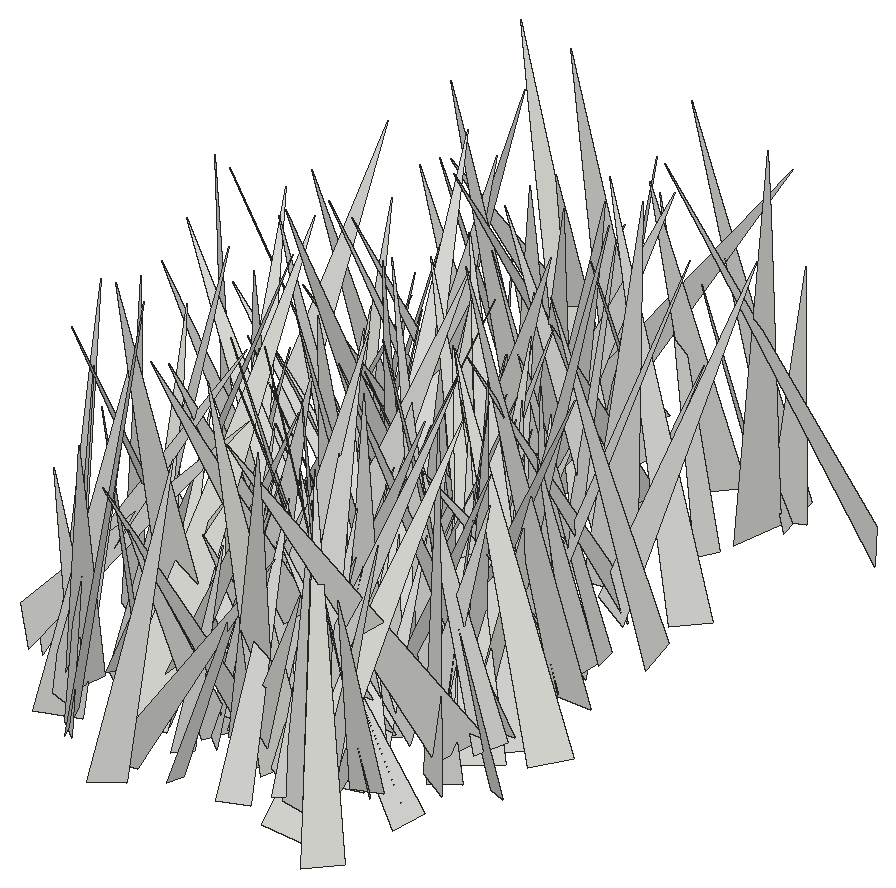
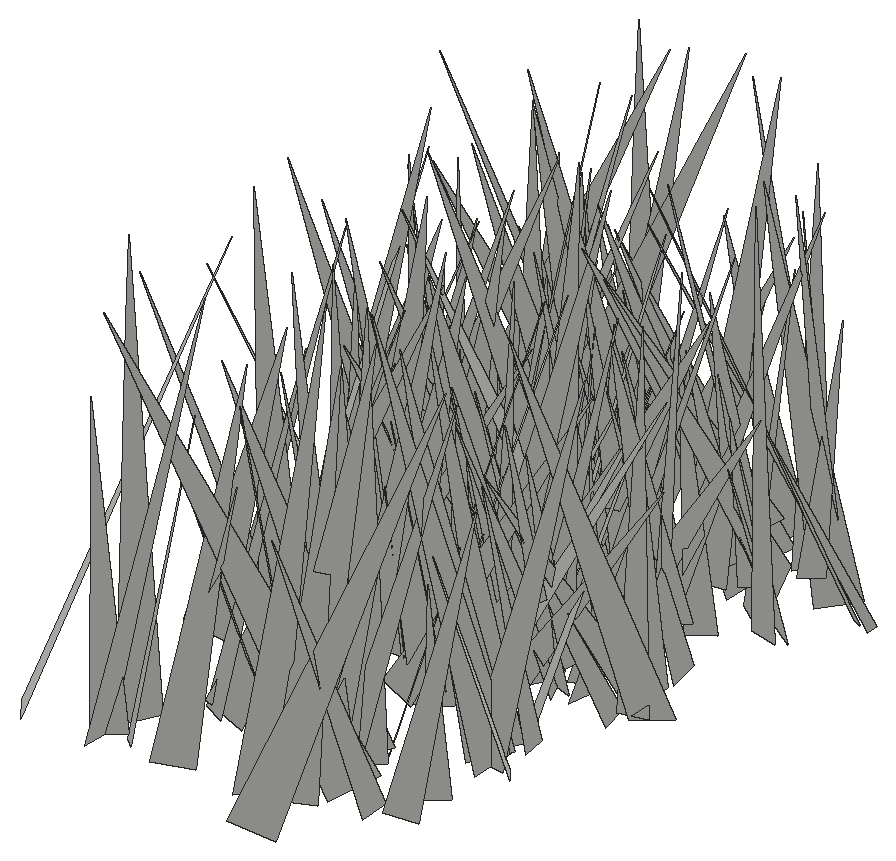
# SketchUp Ruby script. Lengths in inches.
U = 1.inch
M = Sketchup.active_model
def pt(a) = Geom::Point3d.new(a.map { |v| v * U })
def face(e, loops, mat)
  f = e.add_face(loops[0].map { |a| pt(a) })
  loops[1..].each { |l| e.add_face(l.map { |a| pt(a) }).erase! }
  f.material = f.back_material = mat if mat
  f
end
# faces: each face lists its corners as indices into pts; further lists are holes
def faces(e, pts, list, mat = nil) = list.each { |f| face(e, (f[0].is_a?(Array) ? f : [f]).map { |l| l.map { |i| pts[i] } }, mat) }
# xy, xz, yz: faces in a plane at the given z, y or x. An outline is a flat list of corners, or four numbers for a rectangle; further outlines are holes
def ring(l) = l.size == 4 ? [[l[0], l[1]], [l[2], l[1]], [l[2], l[3]], [l[0], l[3]]] : l.each_slice(2).to_a
def flat(e, list, mat, &to3) = list.each { |f| face(e, (f[0].is_a?(Array) ? f : [f]).map { |l| ring(l).map { |u, v| to3.(u, v) } }, mat) }
def xy(e, z, list, mat = nil) = flat(e, list, mat) { |x, y| [x, y, z] }
def xz(e, y, list, mat = nil) = flat(e, list, mat) { |x, z| [x, y, z] }
def yz(e, x, list, mat = nil) = flat(e, list, mat) { |y, z| [x, y, z] }
def lines(e, pts, list) = list.each { |a, b| e.add_line(pt(pts[a]), pt(pts[b])) }
# prism: a flat outline (further loops are holes) pulled along v
def prism(e, loops, v, mat = nil)
  f = face(e, loops, mat); d = Geom::Vector3d.new(v.map { |x| x * U })
  f.pushpull(f.normal.samedirection?(d) ? d.length : -d.length)
end
def box(e, o, s, mat = nil) = prism(e, [[o, [o[0] + s[0], o[1], o[2]], [o[0] + s[0], o[1] + s[1], o[2]], [o[0], o[1] + s[1], o[2]]]], [0, 0, s[2]], mat)
def at(x, y, z, deg = 0) = Geom::Transformation.translation(pt([x, y, z])) * Geom::Transformation.rotation(ORIGIN, Z_AXIS, deg.degrees)
def axes(o, x, y, z) = Geom::Transformation.new([*x, 0, *y, 0, *z, 0, *pt(o).to_a, 1])
def part(name) = M.definitions.add(name)
# library, detail: a bought-in or finely detailed component or shape, given as its bounding box
def library(name, o, s) = part(name).tap { |d| box(d.entities, o, s) }
def detail(e, o, s) = box(e.add_group.entities, o, s)
def put(e, d, t, mat = nil) = e.add_instance(d, t).tap { |i| i.material = mat if mat }
def group(e, t, mat = nil) = e.add_group.tap { |g| g.transformation = t; g.material = mat if mat }.entities
root = M.entities
c1 = part("fur_instance\#9")
p = [[0.8125,0,1.79],[0.67,-0.02,1.48],[0,-0.11,0],[0,0.11,0]]
faces(c1.entities,p,[[0,1,2,3]])
put(root,c1,axes([134.02,205.54,-27.1],[-1.22058,7.14872,1.6543],[7.02907,1.62036,-1.81584],[2.10547,-1.26529,7.02116]))
put(root,c1,axes([134.57,199.46,-27.1],[-2.31612,-6.1908,2.36322],[-6.27799,2.85121,1.3163],[2.12077,1.67923,6.47748]))
put(root,c1,axes([136.18,215.1,-27.1],[1.56838,-4.91392,1.31708],[-4.91027,-1.82266,-0.95305],[-1.33063,0.93404,5.06933]))
put(root,c1,axes([134.63,205.76,-27.1],[-0.27546,-6.0552,1.07535],[-6.00995,0.49341,1.23885],[1.30474,0.99438,5.93351]))
put(root,c1,axes([136.3125,210.85,-27.1],[-0.27695,-6.43694,1.01641],[-6.49492,0.18954,-0.56932],[-0.53231,1.03627,6.4177]))
put(root,c1,axes([135.78,195.63,-27.1],[3.23004,-2.47849,1.2151],[-2.38486,-3.44753,-0.69249],[-1.3899,0.15559,4.01205]))
put(root,c1,axes([138.625,206.86,-27.1],[-4.24155,2.82864,0.08548],[2.61337,3.85608,2.07369],[-1.08573,-1.76881,4.65744]))
put(root,c1,axes([139.25,207.15,-27.1],[-5.24888,-4.54366,0.15791],[-4.36596,4.97023,-2.11085],[-1.26815,1.69482,6.61361]))
put(root,c1,axes([136.17,194.08,-27.1],[2.58836,6.22661,1.98748],[6.38761,-2.86286,0.6503],[-1.38536,-1.56644,6.71174]))
put(root,c1,axes([136.29,196.8,-28.22],[1.50713,3.43781,0.3216],[3.3001,-1.53741,0.96906],[-1.01552,0.10596,3.62641]))
put(root,c1,axes([136.01,213.55,-27.1],[-2.23187,2.81976,1.51549],[3.01775,2.4697,-0.15093],[1.06816,-1.08561,3.59298]))
put(root,c1,axes([136.5,208.49,-27.1],[-3.05725,-3.63504,0.09512],[-3.51202,2.98398,1.15363],[0.94245,-0.67208,4.60753]))
put(root,c1,axes([137.71,200.69,-28.22],[-7.59721,-1.99805,2.32928],[-2.54922,7.5713,-1.81993],[1.70857,2.41215,7.64184]))
put(root,c1,axes([136.1,202.68,-28.22],[4.53301,0.32886,1.81446],[0.26511,-4.88148,0.22244],[-1.82486,0.10775,4.53948]))
put(root,c1,axes([135.27,210.93,-27.1],[2.99336,2.37967,0.42143],[2.41657,-2.95437,-0.48225],[-0.02533,-0.63994,3.79348]))
put(root,c1,axes([137.33,200.68,-27.1],[-3.85678,5.81728,0.33644],[5.7739,3.8696,-0.71896],[0.78484,0.11882,6.94252]))
put(root,c1,axes([136.83,197.25,-27.1],[-1.83169,3.1238,0.57494],[3.14275,1.87858,-0.19441],[0.4602,-0.39568,3.61599]))
put(root,c1,axes([135.76,209.14,-27.1],[4.33952,0.70183,1.00017],[0.70812,-4.45199,0.05164],[-0.99573,-0.10739,4.3956]))
put(root,c1,axes([137.8,204.35,-28.22],[-7.13222,-2.21187,1.52983],[-1.72076,7.08542,2.22194],[2.06682,-1.73369,7.12909]))
put(root,c1,axes([135.28,194.89,-28.22],[4.4224,-5.22883,1.99199],[-5.58659,-4.26873,1.19762],[-0.31423,2.30295,6.7427]))
put(root,c1,axes([135.56,204.58,-27.1],[4.79921,1.03907,0.41248],[0.79797,-4.45725,1.94381],[-0.78297,1.82633,4.50929]))
put(root,c1,axes([132.9375,196.93,-27.1],[5.32286,5.30667,0.20638],[4.93366,-4.8331,-2.97258],[1.96528,-2.23975,6.90343]))
put(root,c1,axes([132.29,197.01,-27.1],[4.7067,5.43888,0.18038],[4.50837,-3.76361,-4.15655],[3.04771,-2.83211,5.87006]))
put(root,c1,axes([137.07,197.03,-28.22],[-3.25628,-4.53556,1.56998],[-4.60157,3.48952,0.53691],[1.36443,0.94415,5.55755]))
put(root,c1,axes([136.23,201.25,-28.22],[5.06172,0.87175,1.3003],[0.68802,-5.19178,0.80241],[-1.40619,0.59773,5.07318]))
put(root,c1,axes([135.62,197.36,-28.22],[-3.45696,-5.56122,4.74392],[-6.59951,4.63089,0.61955],[3.14299,3.60698,6.51874]))
put(root,c1,axes([139.35,199.17,-27.1],[-2.95637,3.32548,0.26078],[3.10336,2.61427,1.84435],[-1.22309,-1.40488,4.04936]))
put(root,c1,axes([138.59,199.73,-28.22],[-3.06964,-6.81398,0.3454],[-6.81954,3.05272,-0.38339],[-0.20825,0.47214,7.46364]))
put(root,c1,axes([137.68,205.73,-27.1],[0.92539,5.82013,0.73982],[5.78512,-1.02986,0.86568],[-0.97656,-0.58571,5.82931]))
put(root,c1,axes([137.36,192.82,-27.1],[3.68214,4.39884,2.0354],[4.4735,-4.06815,0.69917],[-1.86561,-1.07294,5.69378]))
put(root,c1,axes([136.18,196.54,-27.1],[6.68377,2.4417,1.0502],[1.89436,-6.36953,2.75283],[-1.86446,2.28139,6.56175]))
put(root,c1,axes([138.0625,195.86,-27.1],[-5.38629,2.97439,0.98855],[2.72826,5.41671,-1.43257],[1.54299,0.80541,5.98388]))
put(root,c1,axes([138.54,205.72,-27.1],[-6.31827,-0.38458,1.65434],[-0.20418,6.49842,0.73085],[1.68614,-0.65417,6.28763]))
put(root,c1,axes([136.23,204.65,-28.22],[4.0884,0.15219,0.34801],[0.0557,-3.96154,1.07814],[-0.37573,1.0688,3.94662]))
put(root,c1,axes([136.04,195.26,-27.1],[5.72206,-2.67718,0.30846],[-2.55509,-5.6197,-1.37653],[-0.85672,-1.12072,6.16558]))
put(root,c1,axes([135.36,198.06,-27.1],[3.3764,2.66955,0.1135],[2.47122,-3.05035,-1.76859],[1.01611,-1.452,3.92412]))
put(root,c1,axes([138.07,204.73,-27.1],[3.76541,-0.98312,2.37268],[-1.72485,-4.08783,1.04352],[-1.9029,1.75998,3.74912]))
put(root,c1,axes([137.4,198.97,-28.22],[2.1664,-3.98299,1.68795],[-4.30586,-2.16689,0.41322],[-0.41582,1.68731,4.51516]))
put(root,c1,axes([141.62,200.76,-27.1],[-4.54084,5.90887,0.08971],[5.53212,4.21055,2.68494],[-2.07809,-1.7025,6.95162]))
put(root,c1,axes([136.06,210.7,-27.1],[7.69259,-0.4984,1.40276],[-0.64413,-7.77059,0.77146],[-1.3421,0.87272,7.67002]))
put(root,c1,axes([136.43,210.43,-27.1],[4.89354,-4.52263,1.72188],[-4.82903,-4.72322,1.31813],[-0.31551,2.14541,6.53173]))
put(root,c1,axes([137.6,205.68,-27.1],[5.0446,1.96996,1.21492],[1.59207,-5.06819,1.60732],[-1.6799,1.1124,5.17158]))
put(root,c1,axes([138.51,195.8125,-27.1],[-1.52341,4.48001,0.30788],[4.47725,1.54034,-0.26007],[0.34571,-0.20714,4.72479]))
put(root,c1,axes([137.13,193.25,-27.1],[6.97385,3.06548,2.09729],[3.25235,-7.19468,-0.2986],[-1.79388,-1.12684,7.61201]))
put(root,c1,axes([138.26,197.97,-27.1],[1.76512,-7.95634,1.31885],[-8.03843,-1.84494,-0.37166],[-0.65291,1.20466,8.14131]))
put(root,c1,axes([140.49,203.86,-27.1],[-3.6362,-3.51378,0.23491],[-3.4583,3.49912,-1.19165],[-0.6648,1.01649,4.91412]))
put(root,c1,axes([139.24,210.65,-27.1],[-5.93761,-4.29126,0.84113],[-3.95201,5.87307,2.0655],[1.8719,-1.21235,7.02879]))
put(root,c1,axes([138.58,206.69,-27.1],[-1.9531,-3.93926,0.49775],[-3.87343,2.01224,0.72636],[0.87298,0.11511,4.33645]))
put(root,c1,axes([139.25,218.57,-27.1],[4.10096,-6.21113,0.1393],[-5.64172,-3.79303,-3.03306],[-2.60165,-1.56533,6.79681]))
put(root,c1,axes([138.375,203.6,-28.22],[-6.90134,-2.30385,2.57209],[-0.73953,6.60101,3.92832],[3.37291,-3.26662,6.12409]))
put(root,c1,axes([139.78,213.17,-27.1],[-2.67742,-5.68655,1.10676],[-5.79247,2.6077,-0.61446],[-0.09527,1.2623,6.25523]))
put(root,c1,axes([138.95,212.18,-27.1],[-5.78164,-4.6449,0.78576],[-4.06196,5.54542,2.89287],[2.386,-1.8147,6.82889]))
put(root,c1,axes([138.86,194.42,-27.1],[-6.04626,5.73242,0.3376],[5.11125,5.59588,-3.47751],[2.61721,2.31459,7.57131]))
put(root,c1,axes([137.07,215.3,-27.1],[4.6922,-0.3007,0.23761],[-0.32477,-4.66947,0.50417],[-0.20347,0.51889,4.67471]))
put(root,c1,axes([141.125,209.13,-27.1],[-0.84326,-5.89202,0.02664],[-5.53518,0.78295,-2.04363],[-2.01949,0.3143,5.59022]))
put(root,c1,axes([139.04,207.97,-27.1],[0.62863,-8.27068,0.12443],[-8.26435,-0.63324,-0.33804],[-0.34653,0.09834,8.28764]))
put(root,c1,axes([138.26,202.73,-28.22],[-1.07299,-3.39329,1.1863],[-3.30809,1.41653,1.05972],[1.4065,0.74301,3.39746]))
put(root,c1,axes([138.25,206.04,-27.1],[-2.58112,4.19595,2.18678],[4.13957,3.20902,-1.27135],[2.29171,-1.07069,4.75939]))
put(root,c1,axes([140.04,213.76,-27.1],[0.54062,-3.9189,1.26852],[-4.01221,-0.79056,-0.73238],[-0.93225,1.12979,3.88763]))
put(root,c1,axes([137.96,201.32,-27.1],[3.51302,-4.23345,1.0034],[-4.35037,-3.40123,0.88101],[0.05668,1.33409,5.43021]))
put(root,c1,axes([136.41,209.7,-27.1],[0.97454,-6.53217,0.4424],[-5.83998,-0.6651,3.04417],[2.95966,0.83851,5.86106]))
put(root,c1,axes([138.9,206.95,-27.1],[-1.97091,-5.99186,1.73382],[-5.97714,2.33419,1.27215],[1.7839,1.20092,6.17807]))
put(root,c1,axes([141.62,213.34,-27.1],[-4.16616,6.68617,2.08588],[7.00105,3.90518,1.46546],[-0.20279,-2.54114,7.74043]))
put(root,c1,axes([139.93,196.93,-28.22],[2.83348,-4.00549,0.52306],[-3.76222,-2.8494,-1.43972],[-1.47079,-0.42795,4.69039]))
put(root,c1,axes([139.09,192.53,-28.22],[4.47757,-3.00826,2.16701],[-3.51648,-4.52249,0.98776],[-1.1747,2.07164,5.30307]))
put(root,c1,axes([138.02,200.17,-28.22],[2.61538,-3.98544,0.72253],[-3.93735,-2.29982,1.56655],[0.95028,1.43982,4.50221]))
put(root,c1,axes([139.84,203.74,-27.1],[4.20978,2.5999,1.29958],[2.36123,-4.39284,1.13935],[-1.69498,0.33775,4.81493]))
put(root,c1,axes([141,211.54,-27.1],[-1.51779,-7.89387,2.17922],[-8.18213,1.37007,-0.73587],[-0.33897,2.275,8.00471]))
put(root,c1,axes([139.91,206.42,-27.1],[2.79879,-2.29313,0.37979],[-2.08936,-2.74248,-1.16161],[-1.01846,-0.6755,3.42672]))
put(root,c1,axes([140.33,203,-28.22],[-4.47086,-3.62986,0.22446],[-3.11938,4.01034,2.72058],[1.8697,-1.98902,5.07572]))
put(root,c1,axes([140.72,196.44,-27.1],[1.48106,4.37962,0.44895],[4.22706,-1.54701,1.14671],[-1.23071,-0.04293,4.4788]))
put(root,c1,axes([139.71,195.45,-28.22],[3.18405,-1.52738,1.26596],[-1.78098,-3.25535,0.55182],[-0.87386,1.06936,3.48806]))
put(root,c1,axes([137.77,201.68,-28.22],[1.52671,4.77623,1.67607],[4.63081,-0.61106,-2.47682],[2.04382,-2.18327,4.35989]))
put(root,c1,axes([141.28,200.95,-27.1],[-4.99483,-3.69291,1.05885],[-3.66459,5.10128,0.50484],[1.15306,0.21561,6.19121]))
put(root,c1,axes([139.34,216.42,-27.1],[3.47226,-5.91321,0.27335],[-5.89868,-3.48291,-0.41506],[-0.49636,0.02495,6.84473]))
put(root,c1,axes([139.16,208.49,-27.1],[4.92449,-2.5321,0.51516],[-2.43841,-4.92066,-0.87679],[-0.85503,-0.55051,5.46748]))
put(root,c1,axes([140.55,199.76,-28.22],[3.08843,-3.08617,0.55459],[-2.71507,-3.02147,-1.69397],[-1.56857,-0.84658,4.0241]))
put(root,c1,axes([140.7,203.97,-28.22],[-4.31312,-2.31019,0.44376],[-1.59331,3.55068,2.99849],[1.73068,-2.4885,3.8664]))
put(root,c1,axes([140.63,216.55,-27.1],[6.98287,-2.99298,2.96369],[-2.61118,-7.57832,-1.50091],[-3.30502,-0.33623,7.44753]))
put(root,c1,axes([138.16,195.87,-28.22],[6.61677,-1.08212,0.53072],[-1.15649,-6.53431,1.0953],[-0.3394,1.16883,6.6146]))
put(root,c1,axes([142.01,196.9,-28.22],[-0.06223,-5.95217,0.13196],[-5.73579,0.02457,-1.59678],[-1.59576,0.14382,5.73432]))
put(root,c1,axes([139.2,213.22,-27.1],[5.34448,-4.72432,0.68412],[-4.69665,-5.3877,-0.51471],[-0.85369,0.0645,7.11462]))
put(root,c1,axes([141.72,208.02,-27.1],[2.74983,3.97442,1.3241],[3.39736,-3.04242,2.07665],[-2.45097,0.24187,4.36407]))
put(root,c1,axes([140.94,200.93,-28.22],[4.09073,2.15745,2.5023],[2.51133,-4.61824,-0.12369],[-2.14694,-1.2913,4.62314]))
put(root,c1,axes([138.96,201.25,-28.22],[6.44978,-0.00096,0.92482],[0.04605,-6.50733,-0.32793],[-0.92367,-0.33115,6.44144]))
put(root,c1,axes([141.57,202.56,-27.1],[-2.88963,7.72101,0.14725],[7.7077,2.8933,-0.45358],[0.4764,0.02131,8.23153]))
put(root,c1,axes([142.99,201.43,-28.22],[-3.78552,-3.06993,0.30173],[-3.01727,3.58565,-1.37288],[-0.64154,1.25071,4.67652]))
put(root,c1,axes([139.46,203.79,-27.1],[4.72004,-5.82808,0.22381],[-5.80637,-4.72269,-0.52693],[-0.55017,-0.15829,7.48115]))
put(root,c1,axes([139.9,196.65,-28.22],[2.95558,3.83246,1.3061],[4.0436,-2.87668,-0.7093],[-0.20723,-1.47175,4.78749]))
put(root,c1,axes([140.67,202.07,-28.22],[3.99187,0.97882,1.10255],[0.50795,-3.90054,1.62373],[-1.38409,1.39155,3.77579]))
put(root,c1,axes([140.22,207.88,-27.1],[3.37975,2.64749,1.02841],[2.82915,-3.2791,-0.85611],[-0.25046,-1.31446,4.20701]))
put(root,c1,axes([140.38,204.51,-28.22],[4.2696,-0.12633,0.87704],[-0.45536,-4.01534,1.6384],[-0.76014,1.6958,3.94476]))
put(root,c1,axes([138.67,193.68,-28.22],[4.24231,-3.44067,0.07958],[-3.18347,-3.87509,2.16585],[1.3077,1.72835,5.01442]))
put(root,c1,axes([140.98,213.89,-27.1],[-3.67972,-3.6806,3.42599],[-4.33109,4.47676,0.15761],[2.55458,2.28831,5.20214]))
put(root,c1,axes([139.37,212.5,-27.1],[3.36914,-5.54095,2.01408],[-5.73384,-2.5398,2.60427],[1.37175,2.99283,5.93894]))
put(root,c1,axes([139.9,213.02,-27.1],[6.8807,-3.2851,0.24825],[-3.20439,-6.80705,-1.26238],[-0.76512,-1.03432,7.51946]))
put(root,c1,axes([139.33,214.23,-27.1],[-0.1774,-7.7519,1.13116],[-7.17611,0.61466,3.08685],[3.14245,0.96602,7.113]))
put(root,c1,axes([142.15,199.83,-28.22],[3.55115,-1.15094,1.45453],[-0.93925,-3.82501,-0.73353],[-1.59941,-0.30919,3.66022]))
put(root,c1,axes([142.16,202.35,-28.22],[-2.2334,-3.12116,0.78897],[-3.02774,2.36275,0.77617],[1.09405,0.16724,3.75863]))
put(root,c1,axes([141.4,199.49,-28.22],[3.18185,3.17768,0.5905],[3.1987,-3.21478,0.06397],[-0.46337,-0.37158,4.49642]))
put(root,c1,axes([141.42,204.65,-27.1],[3.44436,3.22324,0.28553],[3.18394,-3.45028,0.54084],[-0.57733,0.20181,4.68619]))
put(root,c1,axes([144.41,213.46,-27.1],[-1.51333,-7.7582,0.0595],[-7.60064,1.47034,-1.59746],[-1.5568,0.36304,7.74132]))
put(root,c1,axes([141.85,192.4,-27.1],[4.95008,1.27612,1.12304],[0.89586,-4.89693,1.61571],[-1.4447,1.33589,4.84988]))
put(root,c1,axes([140.2,200.72,-27.1],[-0.29437,7.39176,2.68978],[7.28817,1.26884,-2.68928],[2.95898,-2.3899,6.89148]))
put(root,c1,axes([139.85,208.72,-27.1],[2.97269,-7.01093,0.81561],[-6.80259,-2.60982,2.35986],[1.88234,1.64042,7.24024]))
put(root,c1,axes([142.92,207.26,-27.1],[-0.41482,4.98169,1.32883],[5.15587,0.40286,0.09923],[0.00793,-1.33251,4.99795]))
put(root,c1,axes([140.45,200.28,-28.22],[7.17048,3.0592,0.30714],[3.02615,-7.16002,0.66735],[-0.54355,0.49421,7.76718]))
put(root,c1,axes([142.87,196.68,-28.22],[1.90593,-3.10212,1.28599],[-3.27722,-2.04084,-0.06594],[-0.73267,1.05893,3.64024]))
put(root,c1,axes([145.03,210.4,-27.1],[-6.53044,0.59698,0.86107],[0.69842,6.53195,0.76827],[0.78105,-0.84949,6.51251]))
put(root,c1,axes([144.87,198.13,-27.1],[1.87232,-8.06563,0.81969],[-7.60481,-2.03883,-2.69107],[-2.80947,0.14362,7.83059]))
put(root,c1,axes([138.4375,214.56,-27.1],[5.80573,-6.03364,0.3689],[-5.4436,-4.99608,3.95649],[2.62833,2.98023,7.37953]))
put(root,c1,axes([143.95,195.12,-27.1],[-6.33507,2.2676,3.27677],[3.13305,6.63723,1.4641],[2.46237,-2.61105,6.56746]))
put(root,c1,axes([145.63,203.18,-27.1],[-2.86561,6.0597,1.12131],[6.09085,2.59686,1.53195],[-0.93747,-1.65086,6.5257]))
put(root,c1,axes([143.66,216.875,-27.1],[3.60817,-5.34608,1.25489],[-5.24687,-3.79935,-1.09972],[-1.62036,0.39817,6.35531]))
put(root,c1,axes([143.94,200.88,-27.1],[-6.24986,-4.52728,1.84324],[-4.17742,6.50052,1.80193],[2.5383,-0.44892,7.504]))
put(root,c1,axes([144.45,197.77,-27.1],[1.52611,3.71718,0.33458],[3.41655,-1.5369,1.49113],[-1.50217,0.28087,3.73135]))
put(root,c1,axes([146.59,203.61,-28.22],[-3.87014,-4.65436,0.40491],[-4.4497,3.51193,-2.16136],[-1.42379,1.67578,5.65416]))
put(root,c1,axes([145.77,213.45,-27.1],[-5.65883,0.17912,0.29432],[0.09895,5.4838,-1.43499],[0.33003,1.4272,5.47679]))
put(root,c1,axes([142.23,195.56,-27.1],[0.54119,7.40359,2.44886],[7.61955,0.0202,-1.74498],[1.65906,-2.50787,7.21533]))
put(root,c1,axes([145.62,197.04,-27.1],[-3.60755,4.52257,0.00535],[4.517,3.60276,0.29145],[-0.22451,-0.18592,5.77782]))
put(root,c1,axes([144.18,208.39,-27.1],[2.59525,5.12132,1.23508],[5.09738,-2.78884,0.85303],[-1.33041,-0.69505,5.67763]))
put(root,c1,axes([144.14,192.39,-27.1],[-3.10832,3.75001,0.92239],[3.63037,3.24121,-0.94342],[1.31674,-0.08395,4.77852]))
put(root,c1,axes([145.35,196.65,-27.1],[-4.286,2.05614,0.85108],[2.13965,4.31523,0.34994],[0.6115,-0.68765,4.74078]))
put(root,c1,axes([143.28,201.7,-28.22],[-0.36242,4.3186,2.109],[4.6668,0.82166,-0.88056],[1.14855,-1.97588,4.24338]))
put(root,c1,axes([143.82,201.22,-28.22],[6.07778,0.82962,2.17123],[-0.33597,-5.70106,3.1188],[-2.29992,3.02515,5.28212]))
put(root,c1,axes([144.09,200.08,-28.22],[-2.65217,1.9255,1.58872],[2.09556,2.97695,-0.10973],[1.35655,-0.83418,3.2756]))
put(root,c1,axes([143.84,204.62,-28.22],[-1.06035,5.5551,1.84187],[5.77115,1.30347,-0.60889],[0.97234,-1.67863,5.62252]))
put(root,c1,axes([142.47,195.375,-27.1],[1.32188,-7.44707,0.58602],[-7.30684,-1.16527,1.67389],[1.55318,0.85612,7.37593]))
put(root,c1,axes([146.83,197.09,-28.22],[-5.01465,-5.39389,0.78065],[-5.43536,4.87162,-1.25473],[-0.40033,1.42249,7.25716]))
put(root,c1,axes([144.73,213.55,-27.1],[-3.08937,-5.14938,0.76665],[-5.09175,3.1744,0.80332],[1.08532,0.23487,5.95105]))
put(root,c1,axes([143.16,212.79,-27.1],[2.4928,2.63766,0.46244],[2.65596,-2.35455,-0.88721],[0.34203,-0.94022,3.51911]))
put(root,c1,axes([143.89,204.0625,-27.1],[3.61402,1.40651,0.81578],[1.29809,-3.69316,0.61679],[-0.97915,0.29527,3.8287]))
put(root,c1,axes([147.19,198.87,-28.22],[0.70112,8.01126,1.73468],[7.49163,-1.33281,3.12731],[-3.32639,-1.31314,7.4089]))
put(root,c1,axes([141.74,197.89,-28.22],[6.60673,-3.01857,0.44503],[-3.04917,-6.49303,1.22551],[0.11127,1.29906,7.15953]))
put(root,c1,axes([145.28,201.05,-28.22],[-0.37252,4.33667,0.3989],[4.3129,0.31185,0.63743],[-0.60398,-0.44793,4.30572]))
put(root,c1,axes([142.98,194.55,-27.1],[2.13927,-3.81253,0.27989],[-3.71667,-1.99926,1.17453],[0.89447,0.81104,4.21098]))
put(root,c1,axes([145.25,196.82,-28.22],[-0.09668,3.9627,0.07364],[3.92699,0.08582,0.53775],[-0.5359,-0.08606,3.92724]))
put(root,c1,axes([144.86,205.29,-27.1],[-0.32853,3.96848,1.56907],[4.26678,0.33258,0.05223],[0.07349,-1.56822,3.98171]))
put(root,c1,axes([147.39,206.43,-27.1],[-6.20853,-2.44848,0.56631],[-2.51301,6.03462,-1.45936],[-0.02325,1.56521,6.51238]))
put(root,c1,axes([146.85,195.6,-27.1],[-5.72763,-4.55632,1.57593],[-4.80185,5.61014,-1.23206],[0.43111,1.95337,7.21442]))
put(root,c1,axes([145.82,199.02,-27.1],[-3.34335,-1.51871,0.13226],[-1.40215,3.18862,1.16988],[0.59829,-1.01398,3.48078]))
put(root,c1,axes([144.72,195.1,-28.22],[-1.4542,4.67664,1.33998],[4.76533,1.65076,-0.58976],[0.97884,-1.08869,4.86188]))
put(root,c1,axes([143.33,200.87,-27.1],[5.62442,0.34622,0.61815],[0.22701,-5.5658,1.05184],[-0.67115,1.01884,5.53603]))
put(root,c1,axes([144.09,198.85,-27.1],[1.85268,-6.56464,1.39244],[-6.70428,-1.74747,0.68181],[0.2934,1.52239,6.78691]))
put(root,c1,axes([145.48,193.84,-27.1],[5.43527,-3.00495,4.38513],[-4.48513,-5.95873,1.47596],[-2.85354,3.64214,6.0327]))
put(root,c1,axes([145.67,193.34,-27.1],[1.56469,4.5597,1.40699],[4.65343,-1.78584,0.61247],[-1.05645,-1.11294,4.78163]))
put(root,c1,axes([145.22,197.59,-28.22],[-1.89071,3.52857,0.74513],[3.44423,2.01617,-0.80816],[1.06925,-0.25501,3.92077]))
put(root,c1,axes([146.5,216.95,-27.1],[-7.391,-1.41623,2.02124],[-1.14457,7.62073,1.15434],[2.18657,-0.79801,7.4364]))
put(root,c1,axes([146.24,204.04,-28.22],[-2.34195,3.99616,0.3444],[3.99913,2.35703,-0.15486],[0.30802,-0.21845,4.62925]))
put(root,c1,axes([146.05,195.45,-27.1],[4.40996,1.53054,2.75088],[1.88618,-5.07543,-0.19988],[-2.52036,-1.1203,4.66373]))
put(root,c1,axes([147.6,201.78,-28.22],[-3.99948,7.12267,1.32626],[7.23474,3.8453,1.16596],[-0.38726,-1.72292,8.0851]))
put(root,c1,axes([147.33,200.5,-28.22],[-3.34888,5.66427,0.75226],[5.70524,3.26636,0.80369],[-0.31635,-1.05439,6.53093]))
put(root,c1,axes([145.15,195.24,-28.22],[4.00682,1.30969,1.18737],[1.29487,-4.17692,0.23764],[-1.20352,-0.13365,4.20874]))
put(root,c1,axes([148.1,209.72,-27.1],[-2.07893,6.71015,1.41675],[6.64432,1.60395,2.15305],[-1.69892,-1.93817,6.68674]))
put(root,c1,axes([147.81,196.34,-28.22],[-4.58905,2.11277,0.48874],[2.15665,4.32669,1.54618],[-0.22698,-1.60562,4.80963]))
put(root,c1,axes([145.56,216.625,-27.1],[-3.59225,-3.71334,1.0598],[-3.39845,3.72735,1.54069],[1.83374,-0.36648,4.93148]))
put(root,c1,axes([147.77,200.87,-27.1],[-2.28095,-6.51713,0.89519],[-6.46928,2.05047,-1.55597],[-1.19279,1.34151,6.72716]))
put(root,c1,axes([146.15,201.44,-27.1],[-2.40866,3.6867,1.3913],[3.88066,2.50239,0.08743],[0.68406,-1.21467,4.40293]))
put(root,c1,axes([143.67,200,-28.22],[5.92157,-1.3609,0.111],[-1.36516,-5.91048,0.36315],[-0.02664,0.3788,6.06507]))
put(root,c1,axes([144.78,209.94,-27.1],[2.7668,-7.06079,2.0724],[-7.35623,-2.5972,0.97226],[0.18857,2.28135,7.52095]))
put(root,c1,axes([147.49,199.27,-27.1],[4.76692,-6.38187,0.99404],[-5.33821,-4.5884,-3.85875],[-3.63592,-1.6304,6.96863]))
put(root,c1,axes([145.46,209.7,-27.1],[-5.2335,-6.40482,0.23356],[-5.52847,4.66397,4.0186],[3.24225,-2.38569,7.22925]))
put(root,c1,axes([147.48,192.55,-28.22],[-5.07407,3.61415,0.85454],[3.5922,5.14344,-0.42375],[0.94256,-0.14624,6.2152]))
put(root,c1,axes([148.84,199.33,-28.22],[-4.91979,-5.33902,1.78444],[-5.59743,4.38767,-2.30455],[-0.5985,2.85253,6.88466]))
put(root,c1,axes([147.49,204.07,-27.1],[-3.51582,-2.14374,0.80605],[-2.26912,3.46073,-0.69338],[0.31056,1.01688,4.05904]))
put(root,c1,axes([146.14,205.02,-27.1],[-0.76363,-5.08076,1.72351],[-5.30047,0.98391,0.55201],[0.83046,1.60796,5.10809]))
put(root,c1,axes([145.42,193.35,-28.22],[-2.62249,6.7547,0.84995],[6.3246,2.75431,-2.37468],[2.5195,0.11678,6.84575]))
put(root,c1,axes([144.26,194.44,-27.1],[3.571,6.90444,0.98118],[6.89309,-3.32732,-1.67343],[1.05801,-1.62595,7.59098]))
put(root,c1,axes([147,206.1,-27.1],[-5.34969,-3.46152,0.37635],[-2.75195,4.62606,3.43064],[2.1332,-2.713,5.36954]))
put(root,c1,axes([144.22,202.75,-27.1],[6.32443,-0.86949,0.03215],[-0.87008,-6.31952,0.24926],[0.00213,0.25131,6.37905]))
put(root,c1,axes([145.51,204.7,-27.1],[4.61833,5.37447,0.17353],[5.34108,-4.61135,0.67253],[-0.62281,0.30742,7.05419]))
put(root,c1,axes([145.92,201.84,-28.22],[6.7511,0.38921,2.10678],[0.68602,-6.99103,-0.90679],[-2.02963,-1.06837,6.70124]))
put(root,c1,axes([146.74,193.375,-27.1],[-4.01234,0.85775,1.7856],[0.34464,4.27421,-1.27879],[1.95072,1.00913,3.89863]))
put(root,c1,axes([148.27,203.71,-27.1],[-1.48143,-7.59825,2.03928],[-7.84224,1.26126,-0.99758],[-0.62555,2.18232,7.67677]))
put(root,c1,axes([146.64,201.49,-27.1],[-7.17026,0.40545,3.85637],[-0.86926,7.73252,-2.42922],[3.77894,2.54801,6.75839]))
put(root,c1,axes([146.95,198.59,-28.22],[-2.81459,-5.30869,2.75415],[-5.79641,3.17103,0.18862],[1.47279,2.33491,6.00571]))
put(root,c1,axes([146,199.3125,-27.1],[1.71183,-4.04593,1.56999],[-4.29437,-1.33542,1.2409],[0.62675,1.9005,4.21427]))
put(root,c1,axes([146.51,199.29,-28.22],[5.13574,3.88277,2.0176],[4.11622,-5.34233,-0.19668],[-1.48436,-1.3806,6.4353]))
put(root,c1,axes([148.16,199.89,-27.1],[-4.52682,2.09063,1.69581],[2.46981,4.54531,0.98938],[1.07078,-1.64562,4.88712]))
put(root,c1,axes([146.22,215.33,-27.1],[7.26083,-2.43104,1.92439],[-2.31077,-7.51014,-0.76873],[-2.06726,-0.14373,7.61831]))
put(root,c1,axes([148.54,207.52,-27.1],[-6.39849,-1.36399,1.46981],[-1.16574,6.52941,0.98452],[1.63152,-0.68393,6.46776]))
put(root,c1,axes([146.41,216.54,-27.1],[2.86346,-4.49186,1.0378],[-4.60706,-2.8331,0.44926],[-0.16992,1.11803,5.30796]))
put(root,c1,axes([150.14,200.33,-27.1],[-3.49983,5.63032,0.78088],[5.54982,3.18646,1.89866],[-1.22869,-1.64469,6.35172]))
put(root,c1,axes([147.41,205.39,-27.1],[4.28198,-1.79299,1.3249],[-1.43721,-4.41332,-1.32759],[-1.70429,-0.78312,4.44833]))
put(root,c1,axes([145.6875,208.84,-27.1],[2.61038,6.20008,1.07332],[6.21386,-2.35716,-1.49626],[0.99041,-1.55238,6.55868]))
put(root,c1,axes([146.87,195.48,-27.1],[2.00782,-4.43373,0.05819],[-4.43409,-2.00742,0.0429],[0.01508,0.0707,4.86698]))
put(root,c1,axes([149.46,217.02,-27.1],[-6.65977,-5.09555,0.25994],[-4.96209,6.56797,1.61994],[1.1874,-1.13219,8.22757]))
